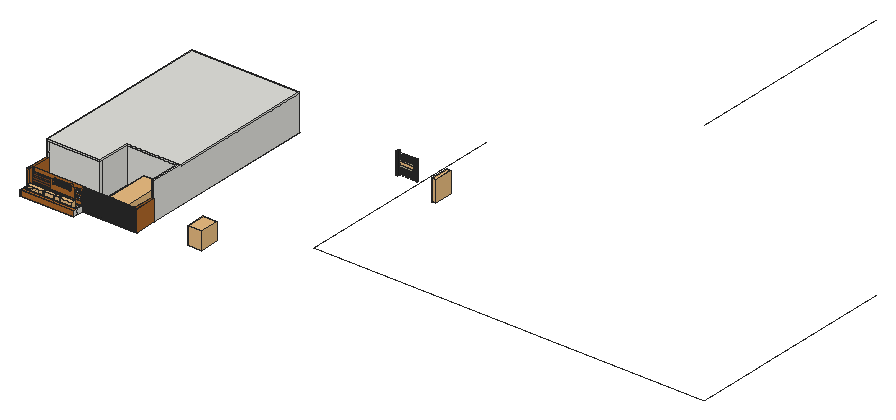
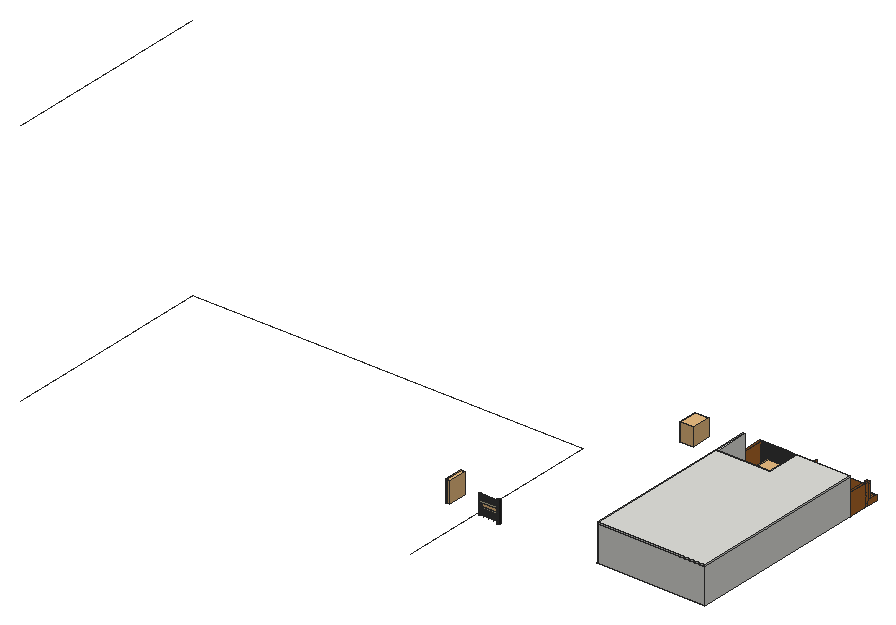
# SketchUp Ruby script. Lengths in inches.
U = 1.inch
M = Sketchup.active_model
def pt(a) = Geom::Point3d.new(a.map { |v| v * U })
def face(e, loops, mat)
  f = e.add_face(loops[0].map { |a| pt(a) })
  loops[1..].each { |l| e.add_face(l.map { |a| pt(a) }).erase! }
  f.material = f.back_material = mat if mat
  f
end
# faces: each face lists its corners as indices into pts; further lists are holes
def faces(e, pts, list, mat = nil) = list.each { |f| face(e, (f[0].is_a?(Array) ? f : [f]).map { |l| l.map { |i| pts[i] } }, mat) }
# xy, xz, yz: faces in a plane at the given z, y or x. An outline is a flat list of corners, or four numbers for a rectangle; further outlines are holes
def ring(l) = l.size == 4 ? [[l[0], l[1]], [l[2], l[1]], [l[2], l[3]], [l[0], l[3]]] : l.each_slice(2).to_a
def flat(e, list, mat, &to3) = list.each { |f| face(e, (f[0].is_a?(Array) ? f : [f]).map { |l| ring(l).map { |u, v| to3.(u, v) } }, mat) }
def xy(e, z, list, mat = nil) = flat(e, list, mat) { |x, y| [x, y, z] }
def xz(e, y, list, mat = nil) = flat(e, list, mat) { |x, z| [x, y, z] }
def yz(e, x, list, mat = nil) = flat(e, list, mat) { |y, z| [x, y, z] }
def lines(e, pts, list) = list.each { |a, b| e.add_line(pt(pts[a]), pt(pts[b])) }
# prism: a flat outline (further loops are holes) pulled along v
def prism(e, loops, v, mat = nil)
  f = face(e, loops, mat); d = Geom::Vector3d.new(v.map { |x| x * U })
  f.pushpull(f.normal.samedirection?(d) ? d.length : -d.length)
end
def box(e, o, s, mat = nil) = prism(e, [[o, [o[0] + s[0], o[1], o[2]], [o[0] + s[0], o[1] + s[1], o[2]], [o[0], o[1] + s[1], o[2]]]], [0, 0, s[2]], mat)
def at(x, y, z, deg = 0) = Geom::Transformation.translation(pt([x, y, z])) * Geom::Transformation.rotation(ORIGIN, Z_AXIS, deg.degrees)
def axes(o, x, y, z) = Geom::Transformation.new([*x, 0, *y, 0, *z, 0, *pt(o).to_a, 1])
def part(name) = M.definitions.add(name)
# library, detail: a bought-in or finely detailed component or shape, given as its bounding box
def library(name, o, s) = part(name).tap { |d| box(d.entities, o, s) }
def detail(e, o, s) = box(e.add_group.entities, o, s)
def put(e, d, t, mat = nil) = e.add_instance(d, t).tap { |i| i.material = mat if mat }
def group(e, t, mat = nil) = e.add_group.tap { |g| g.transformation = t; g.material = mat if mat }.entities
root = M.entities
M.materials.add("Gold Paint").color = [253, 197, 115]
M.materials.add("Metal Black").color = [38, 38, 38]
M.materials.add("Paint").color = [196, 189, 159]
M.materials.add("[Mosaic Hexagonal Tile]").color = [168, 194, 223]
M.materials.add("[Wood Bamboo]").color = [177, 105, 43]
M.materials.add("[Wood Veneer 01]").color = [120, 70, 37]
c1 = library("Lexus+LX570+2016",[436.28,91.76,-4.98],[67.64,149.22,55.27])
c2 = part("Group\#29")
box(c2.entities,[0,0,0],[68,2,2])
c3 = library("Group7\#3",[73.05,1.8125,29.64],[69.11,0.375,12.48])
c4 = library("Group7\#1",[73.1875,1.8,-0.2],[68.8125,0.4,0.4])
c5 = part("Group\#24")
box(c5.entities,[0,0,0],[68,2,2])
c6 = part("Group\#27")
box(c6.entities,[0,0,0],[68,2,2])
c7 = part("Group\#31")
box(c7.entities,[0,0,0],[68,2,2])
c8 = part("Group\#18")
put(c8.entities,c2,at(0,0,8))
put(c8.entities,c2,at(0,0,0))
put(c8.entities,c5,at(0,0,4))
put(c8.entities,c6,at(0,0,12))
g1 = group(c8.entities,at(0,0,16))
box(g1,[0,0,0],[68,2,2])
c9 = library("Group\#15",[0,0,0],[42,3,72])
c10 = part("Metal Gate")
g2 = group(c10.entities,at(66,-0.5,-0.2))
g3 = group(g2,at(-2,0.5,50.2),"Paint")
put(g3,c2,axes([0,0,8],[-1,0,0],[0,1,0],[0,0,1]))
g4 = group(g3,at(0,0,0))
box(g4,[-68,0,0],[68,2,2])
put(g3,c2,axes([0,0,4],[-1,0,0],[0,1,0],[0,0,1]))
g5 = group(g3,at(0,0,12))
box(g5,[-68,0,0],[68,2,2])
put(g3,c2,axes([0,0,16],[-1,0,0],[0,1,0],[0,0,1]))
g6 = group(g2,at(-2,1,42.2),"Paint")
xy(g6,0,[[-68,0,0,2]],"Metal Black")
xy(g6,0.5,[[-67.5,-0.5,0,0]])
xy(g6,5.5,[[-67.5,-0.5,0,0]])
xy(g6,6,[[-68,0,0,2]],"Metal Black")
xz(g6,-0.5,[[-67.5,0.5,0,5.5]])
xz(g6,0,[[-68,0,-68,6,0,6,0,5.5,-67.5,5.5,-67.5,0.5,0,0.5,0,0]],"Metal Black")
xz(g6,2,[[-68,0,0,6]])
yz(g6,-68,[[0,0,2,6]])
yz(g6,-67.5,[[-0.5,0.5,0,5.5]])
yz(g6,0,[[0,0,2,6],[-0.5,0.5,0,5.5]])
g7 = group(g2,at(-2,0.5,4.2),"Paint")
put(g7,c2,axes([0,0,8],[-1,0,0],[0,1,0],[0,0,1]))
put(g7,c2,axes([0,0,0],[-1,0,0],[0,1,0],[0,0,1]))
put(g7,c2,axes([0,0,4],[-1,0,0],[0,1,0],[0,0,1]))
put(g7,c2,axes([0,0,12],[-1,0,0],[0,1,0],[0,0,1]))
put(g7,c2,axes([0,0,16],[-1,0,0],[0,1,0],[0,0,1]))
g8 = group(g2,at(-429.62,-686.26,0.2),"Metal Black")
prism(g8,[[[-72,2,0],[-0.25,2,0],[-0.25,2,72],[-72,2,72]],[[-70,2,70],[-2,2,70],[-2,2,2],[-70,2,2]]],[0,-2,0])
prism(g8,[[[-163.86,4.64,0],[-92.11,4.64,0],[-92.11,4.64,72],[-163.86,4.64,72]],[[-161.86,4.64,70],[-93.86,4.64,70],[-93.86,4.64,2],[-161.86,4.64,2]]],[0,-2,0])
g9 = group(g2,at(-2,1,24.2),"Paint")
xy(g9,0,[[-68,0,0,2]],"Metal Black")
xy(g9,0.5,[[-67.5,-0.5,0,0]])
xy(g9,5.5,[[-67.5,-0.5,0,0]])
xy(g9,6,[[-68,0,0,2]],"Metal Black")
xz(g9,-0.5,[[-67.5,0.5,0,5.5]])
xz(g9,0,[[-68,0,-68,6,0,6,0,5.5,-67.5,5.5,-67.5,0.5,0,0.5,0,0]],"Metal Black")
xz(g9,2,[[-68,0,0,6]])
yz(g9,-68,[[0,0,2,6]])
yz(g9,-67.5,[[-0.5,0.5,0,5.5]])
yz(g9,0,[[0,0,2,6],[-0.5,0.5,0,5.5]])
g10 = group(g2,at(-2,0,25.7),"Gold Paint")
prism(g10,[[[-9,0.5,19],[0,0.5,19],[0,0.5,21],[-11,0.5,21],[-11,0.5,0],[0,0.5,0],[0,0.5,2],[-9,0.5,2]]],[0,-0.5,0])
g11 = group(g2,at(-2,0,29.7),"Gold Paint")
prism(g11,[[[-7.5,0.5,13.5],[-7.5,0.5,-0.5],[0,0.5,-0.5],[0,0.5,1],[-6,0.5,1],[-6,0.5,12],[0,0.5,12],[0,0.5,13.5]]],[0,-0.5,0])
put(g2,c3,axes([72,-0.5,0.2],[-1,0,0],[0,1,0],[0,0,1]),"Gold Paint")
put(g2,c4,axes([72,0.5,0.2],[-1,0,0],[0,1,0],[0,0,1]))
g12 = group(c10.entities,at(-566.96,-688.58,-30.29))
xy(g12,30.29,[[-150.28,-34.98,-150.28,1.58,-140.59,1.58,-140.59,-22.35,32.22,-22.35,32.22,-34.98],[24.92,-22.35,32.22,1.58]])
xy(g12,47.98,[[-150.28,-34.98,32.22,-34.98,32.22,-22.35,-140.59,-22.35,-140.59,1.58,-150.28,1.58],[24.92,-22.35,32.22,1.58]])
xz(g12,-34.98,[[-150.28,30.29,32.22,47.98]])
xz(g12,-22.35,[[-140.59,30.29,24.92,47.98],[24.92,30.29,32.22,47.98]])
xz(g12,1.58,[[-150.28,30.29,-140.59,47.98],[24.92,30.29,32.22,47.98]])
yz(g12,-150.28,[[-34.98,30.29,1.58,47.98]])
yz(g12,-140.59,[[-22.35,30.29,1.58,47.98]])
yz(g12,24.92,[[-22.35,30.29,1.58,47.98]])
yz(g12,32.22,[[-34.98,30.29,-22.35,47.98],[-22.35,30.29,1.58,47.98]])
g13 = group(g12,at(131.31,2.85,30.23),"Paint")
put(g13,c2,axes([0,0,8.24],[1.03,0,0],[0,1.03,0],[0,0,1.03]))
put(g13,c2,axes([0,0,0],[1.03,0,0],[0,1.03,0],[0,0,1.03]))
put(g13,c5,axes([0,0,4.12],[1.03,0,0],[0,1.03,0],[0,0,1.03]))
put(g13,c6,axes([0,0,12.36],[1.03,0,0],[0,1.03,0],[0,0,1.03]))
put(g13,c7,axes([0,0,16.48],[1.03,0,0],[0,1.03,0],[0,0,1.03]))
put(g12,c8,axes([131.31,2.85,46.48],[1.03,0,0],[0,1.03,0],[0,0,1.03]),"Paint")
g14 = group(g12,at(131.31,2.85,60.86),"Paint")
put(g14,c2,axes([0,0,8.24],[1.03,0,0],[0,1.03,0],[0,0,1.03]))
put(g14,c2,axes([0,0,0],[1.03,0,0],[0,1.03,0],[0,0,1.03]))
put(g14,c5,axes([0,0,4.12],[1.03,0,0],[0,1.03,0],[0,0,1.03]))
put(g14,c6,axes([0,0,12.36],[1.03,0,0],[0,1.03,0],[0,0,1.03]))
put(g14,c7,axes([0,0,16.48],[1.03,0,0],[0,1.03,0],[0,0,1.03]))
g15 = group(g12,at(131.31,2.85,82.11),"Paint")
put(g15,c2,axes([0,0,8.24],[1.03,0,0],[0,1.03,0],[0,0,1.03]))
put(g15,c2,axes([0,0,0],[1.03,0,0],[0,1.03,0],[0,0,1.03]))
g16 = group(g15,at(0,0,4.12))
box(g16,[0,0,0],[70.04,2.06,2.06])
put(g15,c6,axes([0,0,12.36],[1.03,0,0],[0,1.03,0],[0,0,1.03]))
g17 = group(g15,at(0,0,16.48))
box(g17,[0,0,0],[70.04,2.06,2.06])
put(g12,c8,axes([39.28,4.46,81.74],[1.03,0,0],[0,1.03,0],[0,0,1.03]),"Paint")
put(g12,c8,axes([39.28,4.46,64.24],[1.03,0,0],[0,1.03,0],[0,0,1.03]),"Paint")
put(g12,c8,axes([39.44,4.46,46.63],[1.03,0,0],[0,1.03,0],[0,0,1.03]),"Paint")
put(g12,c8,axes([39.44,4.46,32.29],[1.03,0,0],[0,1.03,0],[0,0,1.03]),"Paint")
g18 = group(c10.entities,at(144,-2,-6),"Metal Black")
box(g18,[-507.24,-684.76,6],[5.76,5.76,72])
box(g18,[-677.24,-685,6],[5.76,5.76,72])
box(g18,[-598.84,-684.76,6],[5.76,5.76,72])
box(g18,[-592.59,-684.76,6],[5.76,5.76,72])
box(g18,[-585.93,-684.76,6],[5.76,5.76,72])
g19 = group(c10.entities,at(-6,-2,-6),"Metal Black")
box(g19,[0,0,3],[6,6,75])
put(c10.entities,c9,axes([162,-59.72,0],[0.31,0,0],[0,20.74,0],[0,0,1]))
c11 = part("Component\#1")
xy(c11.entities,0,[[0,0,369,0,369,74,360,74,360,9,9,9,9,74,0,74],[9,9,360,9,360,189,184,189,184,74,9,74],[0,74,184,74,184,83,9,83,9,687,360,687,360,198,175.5625,198,175.5625,189,360,189,360,74,369,74,369,696,0,696],[9,83,175,83,175,198,360,198,360,687,9,687],[175,189,175.5625,198]])
xy(c11.entities,120,[[0,74,184,83],[0,83,9,189],[9,83,9,687,360,687,360,198,175.5625,198,175.5625,189,175,189,175,83],[0,189,9,696],[175.5625,189,369,198],
  [360,198,369,696],[9,687,360,696]])
xy(c11.entities,126,[[0,74,184,74,184,189,369,189,369,696,0,696],[360,74,369,189]])
xz(c11.entities,74,[[0,0,9,120],[9,0,184,120],[360,0,369,126],[0,120,184,126]])
xz(c11.entities,83,[[9,0,175,120],[175,0,184,120]])
xz(c11.entities,189,[[175,0,175.5625,120],[175.5625,0,184,120],[184,0,360,120],[184,120,360,126],[360,120,369,126]])
xz(c11.entities,198,[[175.5625,0,360,120]])
xz(c11.entities,687,[[9,0,360,120]])
xz(c11.entities,696,[[0,0,369,120],[0,120,369,126]])
yz(c11.entities,0,[[74,0,696,120],[74,120,696,126]])
yz(c11.entities,9,[[83,0,687,120]])
yz(c11.entities,175,[[83,0,189,120]])
yz(c11.entities,175.5625,[[189,0,198,120]])
yz(c11.entities,184,[[74,0,83,120],[83,0,189,120],[74,120,189,126]])
yz(c11.entities,360,[[74,0,189,126],[198,0,687,120]])
yz(c11.entities,369,[[74,0,696,0,696,120,189,120,189,126,74,126],[189,120,696,126]])
c12 = library("Group\#59",[4.04,-0.51,1.77],[194.11,104.78,93.81])
c13 = part("thar new model")
p = [[0,738.58,0],[0,0,0],[1336.8125,0,0],[1336.8125,738.58,0],[1336.8125,0,845.36],[1336.8125,738.58,845.36]]
lines(c13.entities,p,[[0,1],[1,2],[3,2],[4,5]])
put(c13.entities,c12,axes([-202.48,-229.58,20.39],[0,0.34,0],[-0.4465,0,0],[0,0,0.64]))
c14 = library("Potted flower arrangement",[-0.05,-0.05,0],[59.02,14.54,22.0625])
c15 = part("KUMAR\#2")
xy(c15.entities,0.03,[[6.98,0,6.5,0.03,6.1,0.13,5.77,0.3,5.52,0.53,5.34,0.84,5.21,1.24,5.13,1.73,5.1,2.3125,5.1,5.84,6.43,5.84,6.43,1.84,6.46,1.59,6.57,1.39,6.75,1.27,6.98,1.23,7.21,1.27,7.39,1.41,7.5,1.61,7.54,1.89,7.54,5.84,8.85,5.84,8.85,2.11,8.8,1.43,8.65,0.89,8.41,0.49,8.0625,0.22,7.6,0.05],[0.61,0.16,0.61,5.84,1.9,5.84,1.9,3.17,1.92,3.17,3.14,5.84,4.49,5.84,3.17,2.9375,4.4375,0.16,3.02,0.16,1.92,2.52,1.9,2.52,1.9,0.16],[9.82,0.16,10.43,5.84,12.0625,5.84,12.61,2.68,12.75,3.56,12.9375,4.56,13.1875,5.84,14.85,5.84,15.5,0.16,14.22,0.16,13.88,4.07,13.08,0.16,12.21,0.16,11.375,4.08,11.04,0.16],[[16.03,0.16,17.54,5.84,18.99,5.84,20.5,0.16,19.15,0.16,18.9375,1.11,17.57,1.11,17.35,0.16],[17.81,2.13,18.69,2.13,18.4375,3.37,18.26,4.54,18.24,4.54,18.05,3.35]],[[21.15,0.16,21.15,5.84,22.65,5.84,23.08,5.8125,23.47,5.73,23.8,5.58,24.09,5.375,24.32,5.12,24.49,4.82,24.58,4.48,24.62,4.1,24.57,3.69,24.42,3.3,24.17,2.96,23.83,2.72,24.86,0.16,23.5,0.16,22.46,2.75,22.4375,2.75,22.4375,0.16],[22.4375,3.39,22.8125,3.4375,23.08,3.55,23.24,3.74,23.29,3.99,23.24,4.33,23.1,4.5625,22.83,4.69,22.4375,4.74]]])
c16 = part("SUJAN")
xy(c16.entities,0.03,[[6.94,0,6.47,0.03,6.07,0.13,5.72,0.3,5.43,0.52,5.17,0.85,5,1.24,4.91,1.7,4.88,2.26,4.88,5.82,5.64,5.82,5.64,2.26,5.69,1.6,5.76,1.34,5.89,1.11,6.07,0.91,6.3,0.77,6.59,0.68,6.94,0.65,7.28,0.68,7.57,0.77,7.82,0.91,8,1.11,8.125,1.34,8.2,1.6,8.25,2.25,8.25,5.82,9.01,5.82,9.01,2.26,8.98,1.71,8.89,1.25,8.72,0.85,8.46,0.52,8.17,0.29,7.83,0.13,7.43,0.03],[2.17,0.02,1.59,0.05,1.11,0.14,0.3,0.46,0.3,1.41,0.35,1.41,0.75,1.1,1.2,0.86,1.67,0.72,2.11,0.67,2.67,0.74,2.89,0.82,3.07,0.93,3.31,1.24,3.39,1.625,3.34,1.93,3.22,2.18,3,2.37,2.68,2.5,2.2,2.625,1.65,2.76,1.12,2.95,0.9,3.09,0.71,3.26,0.55,3.47,0.43,3.71,0.36,3.98,0.34,4.3,0.37,4.63,0.47,4.93,0.64,5.21,0.88,5.46,1.17,5.66,1.49,5.81,1.86,5.9,2.26,5.93,2.72,5.9,3.16,5.83,3.57,5.72,3.95,5.56,3.95,4.65,3.9,4.65,3.59,4.88,3.2,5.09,2.76,5.23,2.31,5.27,1.83,5.21,1.45,5.02,1.21,4.74,1.125,4.375,1.17,4.05,1.32,3.8,1.55,3.61,1.875,3.48,2.46,3.34,3.04,3.18,3.55,2.96,3.9,2.64,4.11,2.23,4.18,1.74,4.14,1.41,4.04,1.08,3.875,0.78,3.66,0.53,3.37,0.3125,3.04,0.15,2.65,0.05],[10.56,0.04,10.07,0.07,9.55,0.15,9.55,0.875,9.59,0.875,9.98,0.75,10.46,0.69,10.77,0.71,11.02,0.77,11.2,0.87,11.33,1,11.41,1.17,11.46,1.375,11.49,1.89,11.49,5.22,10.28,5.22,10.28,5.82,12.25,5.82,12.25,1.6,12.22,1.25,12.13,0.9375,11.99,0.67,11.79,0.44,11.54,0.27,11.25,0.14,10.92,0.0625],[[12.75,0.12,14.67,5.82,15.61,5.82,17.53,0.12,16.73,0.12,16.21,1.71,14.03,1.71,13.51,0.12],[14.24,2.36,16,2.36,15.12,5.05]],[18.07,0.12,18.07,5.82,19.15,5.82,21.44,1.31,21.44,5.82,22.15,5.82,22.15,0.12,21.3,0.12,18.78,5.04,18.78,0.12]])
xy(root,0,[[0.513,36.807,1.513,45.807],[1.513,36.807,183.013,45.807],[184.013,36.807,360.513,36.807,360.513,110.807,369.513,110.807,369.513,732.807,1.513,732.807,1.513,110.807,10.513,110.807,10.513,45.807,184.263,45.807],[183.013,36.807,183.013,45.807,183.263,45.807],[183.013,36.807,183.263,45.807,184.013,45.807,184.013,36.807],
  [184.013,36.807,184.013,45.807,184.263,45.807],[360.513,36.807,361.513,110.807],[361.513,36.807,369.513,110.807],[369.513,36.807,370.513,110.807],[0.513,45.807,1.513,110.807],
  [1.513,45.807,9.513,110.807],[9.513,45.807,10.513,110.807],[0.513,110.807,1.513,732.807],[369.513,110.807,370.513,732.807]],"[Wood Bamboo]")
xy(root,17.766,[[9.447,27.566,8.985,27.578,8.986,27.605,9.448,27.592],[10.447,27.566,9.985,27.578,10.225,36.575,10.6875,36.5625],[8.985,27.578,0.273,27.811,0.507,36.563,1.507,36.565,1.507,36.563,9.225,36.574,8.986,27.605],[9.985,27.578,9.448,27.592,9.6875,36.5625,9.273,36.574,10.225,36.575],[9.448,27.592,8.986,27.605,1.273,27.811,1.507,36.563,9.225,36.574,9.273,36.574,9.6875,36.5625],
  [9.448,27.592,8.986,27.605,9.225,36.574,9.225,36.575,9.273,36.574,9.6875,36.5625],[0.507,36.563,0.513,36.807,1.513,36.781,1.507,36.565],[1.507,36.563,1.507,36.565,9.225,36.575,9.225,36.574],[1.507,36.565,1.513,36.781,9.225,36.575],[9.225,36.574,9.225,36.575,9.273,36.574],
  [9.273,36.574,9.225,36.575,10.177,36.576,10.225,36.575],[9.225,36.575,1.513,36.781,1.513,36.807,10.177,36.576]],"[Wood Bamboo]")
xy(root,29.445,[[157.013,36.807,183.013,40.245]],"[Wood Bamboo]")
xy(root,31.318,[[158.886,36.807,181.141,40.245]],"[Wood Bamboo]")
xy(root,48.785,[[82.284,36.807,83.284,45.807],[83.284,36.807,141.284,45.807],[141.284,36.807,142.284,45.807]],"[Wood Bamboo]")
xy(root,60.885,[[158.886,36.807,181.141,40.245]],"[Wood Bamboo]")
xz(root,36.807,[[0.513,0,1.513,64.473],[1.513,0,183.013,0,183.013,29.445,157.013,29.445,157.013,62.757,183.013,62.757,183.013,64.473,142.284,64.473,142.284,48.785,82.284,48.785,82.284,64.473,1.513,64.473],[183.013,0,184.013,64.473],[360.513,0,361.513,72],[361.513,0,369.513,72],
  [369.513,0,370.513,72],[158.886,31.318,181.141,60.885],[82.284,48.785,83.284,64.473],[141.284,48.785,142.284,64.473]],"[Wood Bamboo]")
xz(root,40.245,[[[157.013,29.445,183.013,62.757],[158.886,31.318,181.141,60.885]]],"[Wood Bamboo]")
xz(root,45.807,[[0.513,0,1.513,72],[1.513,0,9.513,72],[9.513,0,10.513,72],[[10.513,0,183.013,72],[82.284,48.785,141.284,64.473]],[183.013,0,184.013,72]],"[Wood Bamboo]")
xz(root,110.807,[[0.513,0,1.513,72.3125],[1.513,0,9.513,72.3125],[9.513,0,10.513,72.3125],[360.513,0,361.513,72],[361.513,0,369.513,72],
  [369.513,0,370.513,72]],"[Wood Bamboo]")
yz(root,0.513,[[36.807,0,45.807,72],[45.807,0,110.807,72.3125]],"[Wood Bamboo]")
yz(root,1.513,[[36.807,0,45.807,72],[45.807,0,110.807,72.3125]],"[Wood Bamboo]")
yz(root,9.513,[[45.807,0,110.807,72.3125]],"[Wood Bamboo]")
yz(root,10.513,[[45.807,0,110.807,72.3125]],"[Wood Bamboo]")
yz(root,82.284,[[[36.807,48.785,45.807,64.473],[41.043,60.074,40.784,60.108,40.543,60.208,40.336,60.367,40.177,60.574,40.077,60.815,40.043,61.074,40.077,61.333,40.177,61.574,40.336,61.781,40.543,61.94,40.784,62.04,41.043,62.074,41.302,62.04,41.543,61.94,41.75,61.781,41.909,61.574,42.009,61.333,42.043,61.074,42.009,60.815,41.909,60.574,41.75,60.367,41.543,60.208,41.302,60.108]]],"[Wood Bamboo]")
yz(root,83.284,[[[36.807,48.785,45.807,64.473],[41.043,60.074,40.784,60.108,40.543,60.208,40.336,60.367,40.177,60.574,40.077,60.815,40.043,61.074,40.077,61.333,40.177,61.574,40.336,61.781,40.543,61.94,40.784,62.04,41.043,62.074,41.302,62.04,41.543,61.94,41.75,61.781,41.909,61.574,42.009,61.333,42.043,61.074,42.009,60.815,41.909,60.574,41.75,60.367,41.543,60.208,41.302,60.108],[41.824,54.178,41.565,54.212,41.324,54.312,41.117,54.471,40.958,54.678,40.858,54.919,40.824,55.178,40.858,55.437,40.958,55.678,41.117,55.885,41.324,56.044,41.565,56.144,41.824,56.178,42.083,56.144,42.324,56.044,42.531,55.885,42.69,55.678,42.79,55.437,42.824,55.178,42.79,54.919,42.69,54.678,42.531,54.471,42.324,54.312,42.083,54.212],[41.658,50.189,41.4,50.223,41.158,50.323,40.951,50.482,40.792,50.689,40.693,50.93,40.658,51.189,40.693,51.448,40.792,51.689,40.951,51.896,41.158,52.055,41.4,52.155,41.658,52.189,41.917,52.155,42.158,52.055,42.366,51.896,42.524,51.689,42.624,51.448,42.658,51.189,42.624,50.93,42.524,50.689,42.366,50.482,42.158,50.323,41.917,50.223]]],"[Wood Bamboo]")
yz(root,141.284,[[[36.807,48.785,45.807,64.473],[41.824,54.178,42.083,54.212,42.324,54.312,42.531,54.471,42.69,54.678,42.79,54.919,42.824,55.178,42.79,55.437,42.69,55.678,42.531,55.885,42.324,56.044,42.083,56.144,41.824,56.178,41.565,56.144,41.324,56.044,41.117,55.885,40.958,55.678,40.858,55.437,40.824,55.178,40.858,54.919,40.958,54.678,41.117,54.471,41.324,54.312,41.565,54.212]]],"[Wood Bamboo]")
yz(root,141.472,[[41.043,60.074,41.302,60.108,41.543,60.208,41.75,60.367,41.909,60.574,42.009,60.815,42.043,61.074,42.009,61.333,41.909,61.574,41.75,61.781,41.543,61.94,41.302,62.04,41.043,62.074,40.784,62.04,40.543,61.94,40.336,61.781,40.177,61.574,40.077,61.333,40.043,61.074,40.077,60.815,40.177,60.574,40.336,60.367,40.543,60.208,40.784,60.108]],"[Wood Bamboo]")
yz(root,141.847,[[41.658,50.189,41.917,50.223,42.158,50.323,42.366,50.482,42.524,50.689,42.624,50.93,42.658,51.189,42.624,51.448,42.524,51.689,42.366,51.896,42.158,52.055,41.917,52.155,41.658,52.189,41.4,52.155,41.158,52.055,40.951,51.896,40.792,51.689,40.693,51.448,40.658,51.189,40.693,50.93,40.792,50.689,40.951,50.482,41.158,50.323,41.4,50.223]],"[Wood Bamboo]")
yz(root,142.284,[[36.807,48.785,45.807,64.473]],"[Wood Bamboo]")
yz(root,142.472,[[41.043,60.074,41.302,60.108,41.543,60.208,41.75,60.367,41.909,60.574,42.009,60.815,42.043,61.074,42.009,61.333,41.909,61.574,41.75,61.781,41.543,61.94,41.302,62.04,41.043,62.074,40.784,62.04,40.543,61.94,40.336,61.781,40.177,61.574,40.077,61.333,40.043,61.074,40.077,60.815,40.177,60.574,40.336,60.367,40.543,60.208,40.784,60.108]],"[Wood Bamboo]")
yz(root,157.013,[[36.807,29.445,40.245,62.757]],"[Wood Bamboo]")
yz(root,158.886,[[36.807,31.318,40.245,60.885]],"[Wood Bamboo]")
yz(root,181.141,[[36.807,31.318,40.245,60.885]],"[Wood Bamboo]")
yz(root,183.013,[[36.807,0,36.807,29.445,40.245,29.445,40.245,62.757,36.807,62.757,36.807,64.473,27.807,64.473,27.807,72,45.807,72,45.807,0],[36.807,29.445,40.245,62.757]],"[Wood Bamboo]")
yz(root,184.013,[[36.807,0,36.807,64.473,27.807,64.473,27.807,72,45.807,72,45.807,0]],"[Wood Bamboo]")
yz(root,360.513,[[36.807,0,110.807,72]],"[Wood Bamboo]")
yz(root,361.513,[[36.807,0,110.807,72]],"[Wood Bamboo]")
yz(root,369.513,[[36.807,0,110.807,72]],"[Wood Bamboo]")
yz(root,370.513,[[36.807,0,110.807,72]],"[Wood Bamboo]")
p = [[9.447,27.566,72],[0.273,27.811,72],[0.273,27.811,64.473],[0.273,27.811,17.766],[8.985,27.578,17.766],[9.447,27.566,17.766],
  [1.393,27.807,72],[1.273,27.811,72],[1.273,27.811,64.473],[1.273,27.811,17.766],[8.986,27.605,17.766],[9.448,27.592,17.766],
  [9.985,27.578,17.766],[10.447,27.566,17.766],[10.447,27.566,72],[9.448,27.592,72],[9.6875,36.5625,48.169],[9.6875,36.5625,52.953],
  [9.6875,36.5625,59.391],[9.6875,36.5625,72],[9.454,27.807,72],[9.6875,36.5625,17.766],[9.6875,36.5625,33.607],[9.6875,36.5625,40.669],
  [10.6875,36.5625,59.391],[10.6875,36.5625,72],[10.454,27.807,72],[10.6875,36.5625,17.766],[10.6875,36.5625,33.607],[10.6875,36.5625,40.669],
  [10.6875,36.5625,48.169],[10.6875,36.5625,52.953],[0.513,36.807,64.473],[0.513,36.807,17.766],[0.507,36.563,17.766],[1.513,36.807,64.473],
  [1.513,36.807,17.766],[1.513,36.781,17.766],[1.507,36.565,17.766],[1.507,36.563,17.766],[183.013,36.807,17.766],[183.013,36.807,28.268],
  [70.282,36.657,28.268],[0,36.5625,28.268],[0,36.5625,17.766],[9.225,36.575,17.766],[10.177,36.576,17.766],[0.513,36.807,72],
  [1.513,36.781,72],[9.273,36.574,17.766],[10.225,36.575,17.766],[184.013,36.807,17.766],[184.013,36.807,28.268],[71.282,36.657,28.268],
  [1,36.5625,28.268],[1,36.5625,17.766],[9.225,36.574,17.766],[1.513,36.807,72],[10.694,36.657,28.268],[10.694,36.807,64.473],
  [9.694,36.807,64.473],[9.694,36.657,28.268],[70.282,36.788,59.718],[70.282,36.807,64.473],[71.282,36.807,64.473],[71.282,36.788,59.718],
  [83.284,41.158,50.323],[83.284,41.4,50.223],[141.847,41.4,50.223],[141.847,41.158,50.323],[83.284,41.658,50.189],[141.847,41.658,50.189],
  [83.284,41.917,50.223],[141.847,41.917,50.223],[83.284,42.158,50.323],[141.847,42.158,50.323],[83.284,40.951,50.482],[141.847,40.951,50.482],
  [83.284,42.366,50.482],[141.847,42.366,50.482],[83.284,40.792,50.689],[141.847,40.792,50.689],[83.284,42.524,50.689],[141.847,42.524,50.689],
  [83.284,40.693,50.93],[141.847,40.693,50.93],[83.284,42.624,50.93],[141.847,42.624,50.93],[83.284,40.658,51.189],[141.847,40.658,51.189],
  [83.284,42.658,51.189],[141.847,42.658,51.189],[83.284,40.693,51.448],[141.847,40.693,51.448],[83.284,42.624,51.448],[141.847,42.624,51.448],
  [83.284,40.792,51.689],[141.847,40.792,51.689],[83.284,42.524,51.689],[141.847,42.524,51.689],[83.284,40.951,51.896],[141.847,40.951,51.896],
  [83.284,42.366,51.896],[141.847,42.366,51.896],[83.284,41.158,52.055],[141.847,41.158,52.055],[83.284,42.158,52.055],[141.847,42.158,52.055],
  [83.284,41.4,52.155],[141.847,41.4,52.155],[83.284,41.917,52.155],[141.847,41.917,52.155],[83.284,41.658,52.189],[141.847,41.658,52.189],
  [83.284,41.324,54.312],[83.284,41.565,54.212],[141.284,41.565,54.212],[141.284,41.324,54.312],[83.284,41.824,54.178],[141.284,41.824,54.178],
  [83.284,42.083,54.212],[141.284,42.083,54.212],[83.284,42.324,54.312],[141.284,42.324,54.312],[83.284,41.117,54.471],[141.284,41.117,54.471],
  [83.284,42.531,54.471],[141.284,42.531,54.471],[83.284,40.958,54.678],[141.284,40.958,54.678],[83.284,42.69,54.678],[141.284,42.69,54.678],
  [83.284,40.858,54.919],[141.284,40.858,54.919],[83.284,42.79,54.919],[141.284,42.79,54.919],[83.284,40.824,55.178],[141.284,40.824,55.178],
  [83.284,42.824,55.178],[141.284,42.824,55.178],[83.284,40.858,55.437],[141.284,40.858,55.437],[83.284,42.79,55.437],[141.284,42.79,55.437],
  [83.284,40.958,55.678],[141.284,40.958,55.678],[83.284,42.69,55.678],[141.284,42.69,55.678],[83.284,41.117,55.885],[141.284,41.117,55.885],
  [83.284,42.531,55.885],[141.284,42.531,55.885],[83.284,41.324,56.044],[141.284,41.324,56.044],[83.284,42.324,56.044],[141.284,42.324,56.044],
  [83.284,41.565,56.144],[141.284,41.565,56.144],[83.284,42.083,56.144],[141.284,42.083,56.144],[83.284,41.824,56.178],[141.284,41.824,56.178],
  [82.284,40.784,60.108],[83.284,40.784,60.108],[83.284,40.543,60.208],[82.284,40.543,60.208],[141.472,40.784,60.108],[141.472,40.543,60.208],
  [142.472,40.784,60.108],[142.472,40.543,60.208],[82.284,41.043,60.074],[83.284,41.043,60.074],[141.472,41.043,60.074],[142.472,41.043,60.074],
  [82.284,41.302,60.108],[83.284,41.302,60.108],[141.472,41.302,60.108],[142.472,41.302,60.108],[82.284,41.543,60.208],[83.284,41.543,60.208],
  [141.472,41.543,60.208],[142.472,41.543,60.208],[83.284,40.336,60.367],[82.284,40.336,60.367],[141.472,40.336,60.367],[142.472,40.336,60.367],
  [82.284,41.75,60.367],[83.284,41.75,60.367],[141.472,41.75,60.367],[142.472,41.75,60.367],[83.284,40.177,60.574],[82.284,40.177,60.574],
  [141.472,40.177,60.574],[142.472,40.177,60.574],[82.284,41.909,60.574],[83.284,41.909,60.574],[141.472,41.909,60.574],[142.472,41.909,60.574],
  [83.284,40.077,60.815],[82.284,40.077,60.815],[141.472,40.077,60.815],[142.472,40.077,60.815],[82.284,42.009,60.815],[83.284,42.009,60.815],
  [141.472,42.009,60.815],[142.472,42.009,60.815],[83.284,40.043,61.074],[82.284,40.043,61.074],[141.472,40.043,61.074],[142.472,40.043,61.074],
  [82.284,42.043,61.074],[83.284,42.043,61.074],[141.472,42.043,61.074],[142.472,42.043,61.074],[83.284,40.077,61.333],[82.284,40.077,61.333],
  [141.472,40.077,61.333],[142.472,40.077,61.333],[82.284,42.009,61.333],[83.284,42.009,61.333],[141.472,42.009,61.333],[142.472,42.009,61.333],
  [83.284,40.177,61.574],[82.284,40.177,61.574],[141.472,40.177,61.574],[142.472,40.177,61.574],[82.284,41.909,61.574],[83.284,41.909,61.574],
  [141.472,41.909,61.574],[142.472,41.909,61.574],[83.284,40.336,61.781],[82.284,40.336,61.781],[141.472,40.336,61.781],[142.472,40.336,61.781],
  [82.284,41.75,61.781],[83.284,41.75,61.781],[141.472,41.75,61.781],[142.472,41.75,61.781],[83.284,40.543,61.94],[82.284,40.543,61.94],
  [141.472,40.543,61.94],[142.472,40.543,61.94],[82.284,41.543,61.94],[83.284,41.543,61.94],[141.472,41.543,61.94],[142.472,41.543,61.94],
  [83.284,40.784,62.04],[82.284,40.784,62.04],[141.472,40.784,62.04],[142.472,40.784,62.04],[82.284,41.302,62.04],[83.284,41.302,62.04],
  [141.472,41.302,62.04],[142.472,41.302,62.04],[83.284,41.043,62.074],[82.284,41.043,62.074],[141.472,41.043,62.074],[142.472,41.043,62.074],
  [70.282,36.788,48.496],[70.282,36.788,40.996],[70.282,36.788,33.933],[70.282,36.788,53.28],[71.282,36.788,48.496],[71.282,36.788,33.933],
  [71.282,36.788,40.996],[71.282,36.788,53.28]]
faces(root,p,[[0,1,2,3,4,5],[6,7,8,9,10,11,12,13,14,15],[16,17,18,19,20,15,0,5,11,21,22,23],[24,25,26,14,13,27,28,29,30,31],[32,33,34,3,2],[35,36,37,38,39,9,8],[40,41,42,43,44,34,38,45,46],[32,47,48,19,18,17,16,23,22,21,49,45,37,33],
  [50,51,52,53,54,55,39,56,49],[57,25,24,31,30,29,28,27,50,46,36,35],[58,59,60,61],[64,63,62,42,53,65],[66,67,68,69],[67,70,71,68],[70,72,73,71],[72,74,75,73],
  [76,66,69,77],[74,78,79,75],[80,76,77,81],[78,82,83,79],[84,80,81,85],[82,86,87,83],[88,84,85,89],[86,90,91,87],
  [92,88,89,93],[90,94,95,91],[96,92,93,97],[94,98,99,95],[100,96,97,101],[98,102,103,99],[104,100,101,105],[102,106,107,103],
  [108,104,105,109],[106,110,111,107],[112,108,109,113],[110,112,113,111],[114,115,116,117],[115,118,119,116],[118,120,121,119],[120,122,123,121],
  [124,114,117,125],[122,126,127,123],[128,124,125,129],[126,130,131,127],[132,128,129,133],[130,134,135,131],[136,132,133,137],[134,138,139,135],
  [140,136,137,141],[138,142,143,139],[144,140,141,145],[142,146,147,143],[148,144,145,149],[146,150,151,147],[152,148,149,153],[150,154,155,151],
  [156,152,153,157],[154,158,159,155],[160,156,157,161],[158,160,161,159],[162,163,164,165],[163,166,167,164],[166,168,169,167],[170,171,163,162],
  [171,172,166,163],[172,173,168,166],[174,175,171,170],[175,176,172,171],[176,177,173,172],[178,179,175,174],[179,180,176,175],[180,181,177,176],
  [165,164,182,183],[164,167,184,182],[167,169,185,184],[186,187,179,178],[187,188,180,179],[188,189,181,180],[182,190,191,183],[182,184,192,190],
  [185,193,192,184],[186,194,195,187],[195,196,188,187],[188,196,197,189],[190,198,199,191],[190,192,200,198],[193,201,200,192],[194,202,203,195],
  [203,204,196,195],[196,204,205,197],[198,206,207,199],[198,200,208,206],[201,209,208,200],[202,210,211,203],[211,212,204,203],[204,212,213,205],
  [206,214,215,207],[206,208,216,214],[209,217,216,208],[210,218,219,211],[219,220,212,211],[212,220,221,213],[214,222,223,215],[214,216,224,222],
  [217,225,224,216],[218,226,227,219],[227,228,220,219],[220,228,229,221],[222,230,231,223],[222,224,232,230],[225,233,232,224],[226,234,235,227],
  [235,236,228,227],[228,236,237,229],[231,230,238,239],[230,232,240,238],[232,233,241,240],[242,243,235,234],[243,244,236,235],[244,245,237,236],
  [239,238,246,247],[238,240,248,246],[240,241,249,248],[250,251,243,242],[251,252,244,243],[252,253,245,244],[247,246,254,255],[246,248,256,254],
  [248,249,257,256],[255,254,251,250],[254,256,252,251],[256,257,253,252]],"[Wood Bamboo]")
faces(root,p,[[42,62,63,59,58]],"[Wood Veneer 01]")
lines(root,p,[[18,62],[16,258],[23,259],[22,260],[17,261],[30,262],[28,263],[29,264],[31,265],[24,65]])
put(root,c1,at(-191.84,-17.93,0))
put(root,c10,at(717.76,723.81,0))
put(root,c10,at(717.24,723.5625,0.08),"[Wood Bamboo]")
put(root,c11,at(0.51,36.81,-0.25))
put(root,c13,at(791.33,267.99,0))
put(root,c14,at(10.86,12.92,9.27))
put(root,c14,at(65.55,12.92,9.27))
put(root,c14,at(106.11,12.92,9.27))
put(root,c14,at(10.86,12.92,9.9375))
put(root,c15,axes([158.56,36.81,37.85],[0.86,0,0],[0,0,0.86],[0,-0.86,0]),"[Mosaic Hexagonal Tile]")
put(root,c16,axes([158.6,36.81,52.68],[1,0,0],[0,0,1],[0,-1,0]))
